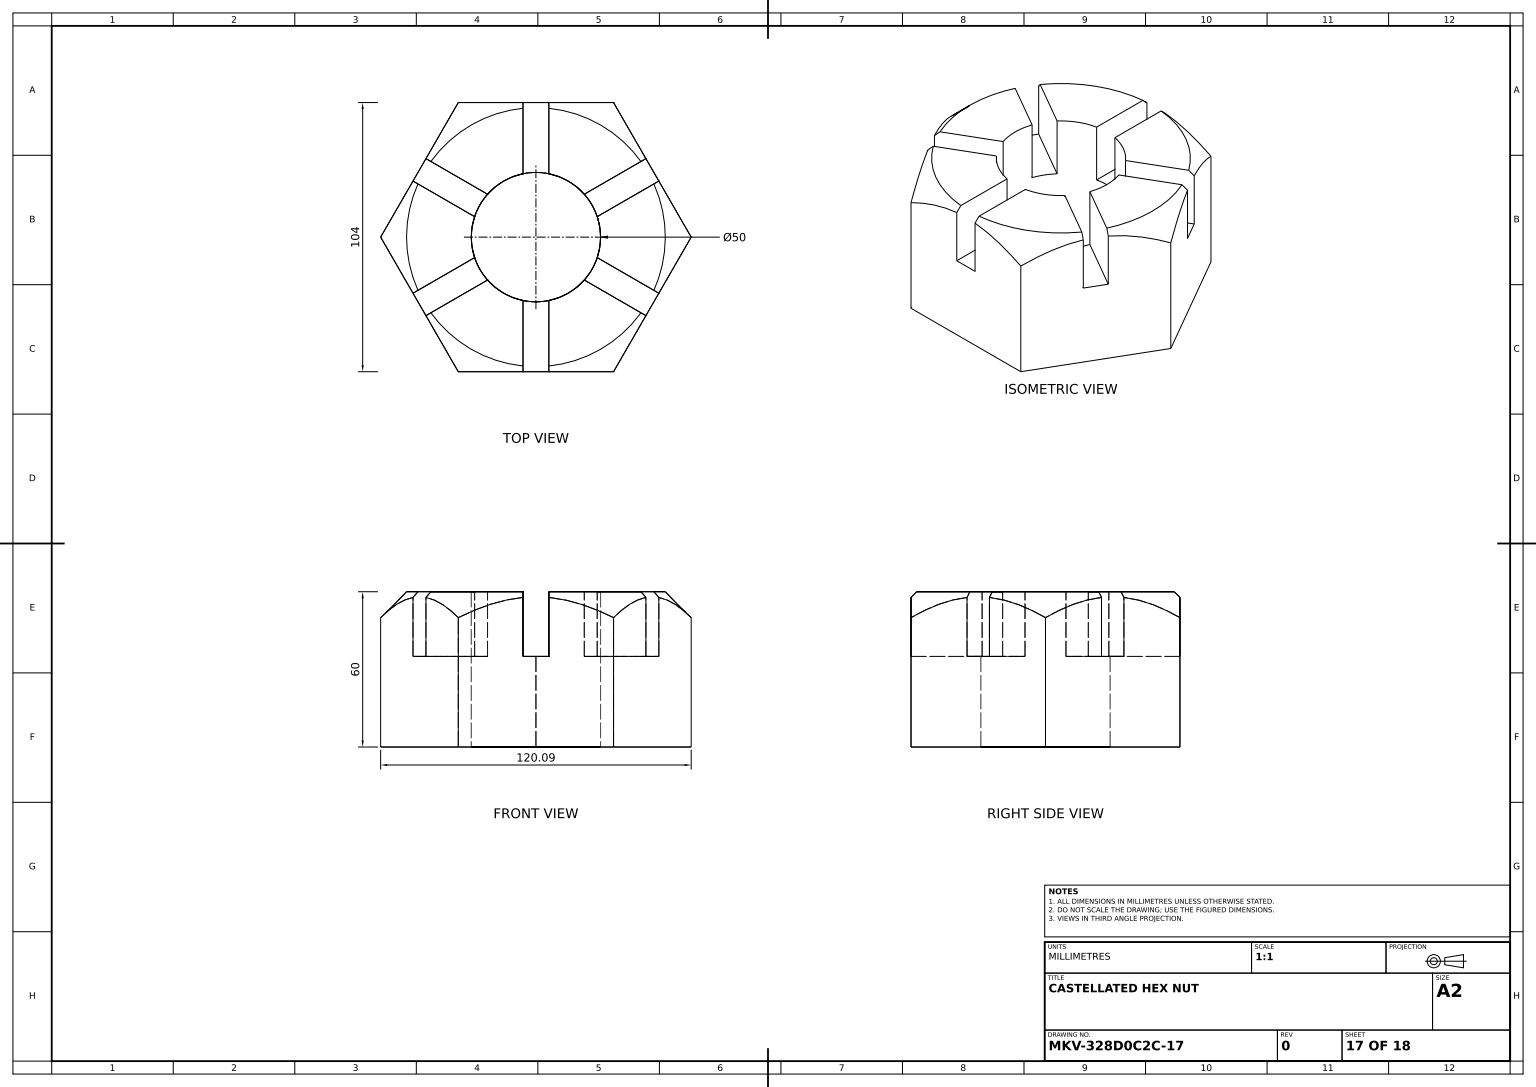
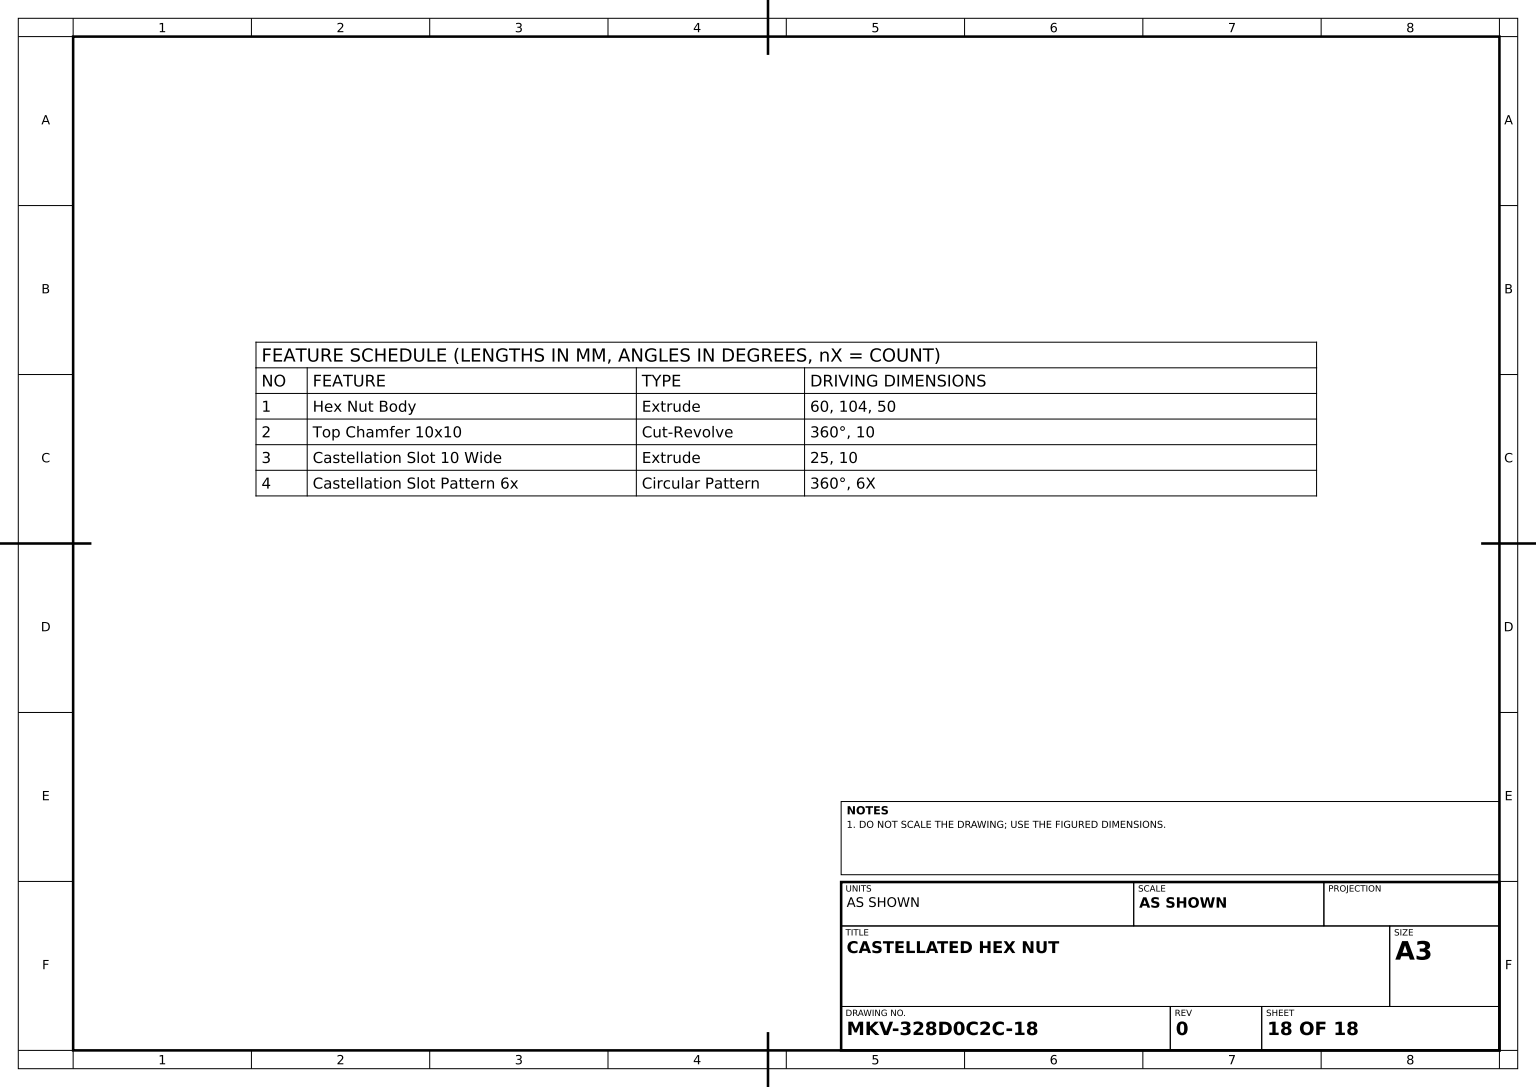
ISO-10303-21;
HEADER;
FILE_DESCRIPTION((''),'2;1');
FILE_NAME('','',(''),(''),'','','');
FILE_SCHEMA(('AUTOMOTIVE_DESIGN'));
ENDSEC;
DATA;
#1=APPLICATION_CONTEXT('');
#2=PRODUCT_CONTEXT('',#1,'mechanical');
#3=PRODUCT('','','',(#2));
#4=PRODUCT_DEFINITION_FORMATION('','',#3);
#5=PRODUCT_DEFINITION_CONTEXT('',#1,'design');
#6=PRODUCT_DEFINITION('','',#4,#5);
#7=PRODUCT_DEFINITION_SHAPE('','',#6);
#8=(LENGTH_UNIT()NAMED_UNIT(*)SI_UNIT(.MILLI.,.METRE.));
#9=(NAMED_UNIT(*)PLANE_ANGLE_UNIT()SI_UNIT($,.RADIAN.));
#10=(NAMED_UNIT(*)SI_UNIT($,.STERADIAN.)SOLID_ANGLE_UNIT());
#11=UNCERTAINTY_MEASURE_WITH_UNIT(LENGTH_MEASURE(1.E-05),#8,'distance_accuracy_value','');
#12=(GEOMETRIC_REPRESENTATION_CONTEXT(3)GLOBAL_UNCERTAINTY_ASSIGNED_CONTEXT((#11))GLOBAL_UNIT_ASSIGNED_CONTEXT((#8,#9,#10))REPRESENTATION_CONTEXT('',''));
#13=CARTESIAN_POINT('',(18.713203,-25.,16.577576));
#14=VERTEX_POINT('',#13);
#15=CARTESIAN_POINT('',(42.533321,-25.,30.330127));
#16=VERTEX_POINT('',#15);
#17=DIRECTION('',(0.866025404,0.,0.5));
#18=VECTOR('',#17,1000.);
#19=LINE('',#13,#18);
#20=EDGE_CURVE('',#14,#16,#19,.T.);
#21=ORIENTED_EDGE('',*,*,#20,.F.);
#22=CARTESIAN_POINT('',(18.713203,0.,16.577576));
#23=VERTEX_POINT('',#22);
#24=DIRECTION('',(0.,1.,0.));
#25=VECTOR('',#24,1000.);
#26=LINE('',#13,#25);
#27=EDGE_CURVE('',#14,#23,#26,.T.);
#28=ORIENTED_EDGE('',*,*,#27,.T.);
#29=CARTESIAN_POINT('',(40.622889,0.,29.227139));
#30=VERTEX_POINT('',#29);
#31=LINE('',#22,#18);
#32=EDGE_CURVE('',#23,#30,#31,.T.);
#33=ORIENTED_EDGE('',*,*,#32,.T.);
#34=CARTESIAN_POINT('',(42.533321,-2.195404,30.330127));
#35=VERTEX_POINT('',#34);
#36=CARTESIAN_POINT('',(41.896575,-1.463528,29.962501));
#37=CARTESIAN_POINT('',(41.259767,-0.731723,29.59484));
#38=B_SPLINE_CURVE_WITH_KNOTS('',3,(#34,#36,#37,#29),.UNSPECIFIED.,.F.,.F.,(4,4),(0.000000326,0.003112581),.UNSPECIFIED.);
#39=EDGE_CURVE('',#35,#30,#38,.T.);
#40=ORIENTED_EDGE('',*,*,#39,.F.);
#41=LINE('',#15,#25);
#42=EDGE_CURVE('',#16,#35,#41,.T.);
#43=ORIENTED_EDGE('',*,*,#42,.F.);
#44=EDGE_LOOP('',(#21,#28,#33,#40,#43));
#45=FACE_OUTER_BOUND('',#44,.T.);
#46=DIRECTION('',(-0.5,0.,0.866025404));
#47=AXIS2_PLACEMENT_3D('',#13,#46,#17);
#48=PLANE('',#47);
#49=ADVANCED_FACE('',(#45),#48,.F.);
#50=CARTESIAN_POINT('',(30.022214,-10.,52.));
#51=VERTEX_POINT('',#50);
#52=CARTESIAN_POINT('',(32.004718,-8.017496,48.566202));
#53=CARTESIAN_POINT('',(34.025227,-6.287322,45.066578));
#54=CARTESIAN_POINT('',(38.18079,-3.587487,37.868931));
#55=CARTESIAN_POINT('',(40.316146,-2.619826,34.170387));
#56=B_SPLINE_CURVE_WITH_KNOTS('',3,(#50,#52,#53,#54,#55,#34),.UNSPECIFIED.,.F.,.F.,(4,2,4),(0.000000254,0.013105191,0.026210128),.UNSPECIFIED.);
#57=EDGE_CURVE('',#51,#35,#56,.T.);
#58=ORIENTED_EDGE('',*,*,#57,.F.);
#59=CARTESIAN_POINT('',(30.022214,-60.,52.));
#60=VERTEX_POINT('',#59);
#61=LINE('',#59,#25);
#62=EDGE_CURVE('',#60,#51,#61,.T.);
#63=ORIENTED_EDGE('',*,*,#62,.F.);
#64=CARTESIAN_POINT('',(60.044428,-60.,0.));
#65=VERTEX_POINT('',#64);
#66=DIRECTION('',(0.5,0.,-0.866025404));
#67=VECTOR('',#66,1000.);
#68=LINE('',#59,#67);
#69=EDGE_CURVE('',#60,#65,#68,.T.);
#70=ORIENTED_EDGE('',*,*,#69,.T.);
#71=CARTESIAN_POINT('',(60.044428,-10.,0.));
#72=VERTEX_POINT('',#71);
#73=LINE('',#64,#25);
#74=EDGE_CURVE('',#65,#72,#73,.T.);
#75=ORIENTED_EDGE('',*,*,#74,.T.);
#76=CARTESIAN_POINT('',(47.533321,-2.195404,21.669873));
#77=VERTEX_POINT('',#76);
#78=CARTESIAN_POINT('',(48.617849,-2.403009,19.791415));
#79=CARTESIAN_POINT('',(49.694995,-2.743391,17.925744));
#80=CARTESIAN_POINT('',(51.300659,-3.434777,15.144652));
#81=CARTESIAN_POINT('',(51.834208,-3.695312,14.220518));
#82=CARTESIAN_POINT('',(52.898163,-4.272921,12.377694));
#83=CARTESIAN_POINT('',(53.428213,-4.589936,11.45962));
#84=CARTESIAN_POINT('',(55.000546,-5.610311,8.73626));
#85=CARTESIAN_POINT('',(56.029879,-6.385229,6.953403));
#86=CARTESIAN_POINT('',(58.058316,-8.086554,3.440047));
#87=CARTESIAN_POINT('',(59.057416,-9.012988,1.709555));
#88=B_SPLINE_CURVE_WITH_KNOTS('',3,(#76,#78,#79,#80,#81,#82,#83,#84,#85,#86,#87,#71),.UNSPECIFIED.,.F.,.F.,(4,2,2,2,2,4),(0.036078749,0.042565008,0.045808138,0.049051268,0.055537527,0.062023787),.UNSPECIFIED.);
#89=EDGE_CURVE('',#77,#72,#88,.T.);
#90=ORIENTED_EDGE('',*,*,#89,.F.);
#91=CARTESIAN_POINT('',(47.533321,-25.,21.669873));
#92=VERTEX_POINT('',#91);
#93=LINE('',#91,#25);
#94=EDGE_CURVE('',#92,#77,#93,.T.);
#95=ORIENTED_EDGE('',*,*,#94,.F.);
#96=LINE('',#91,#67);
#97=EDGE_CURVE('',#16,#92,#96,.T.);
#98=ORIENTED_EDGE('',*,*,#97,.F.);
#99=ORIENTED_EDGE('',*,*,#42,.T.);
#100=EDGE_LOOP('',(#58,#63,#70,#75,#90,#95,#98,#99));
#101=FACE_OUTER_BOUND('',#100,.T.);
#102=AXIS2_PLACEMENT_3D('',#59,#17,#66);
#103=PLANE('',#102);
#104=ADVANCED_FACE('',(#101),#103,.T.);
#105=CARTESIAN_POINT('',(23.713203,-25.,-7.917322));
#106=VERTEX_POINT('',#105);
#107=CARTESIAN_POINT('',(47.533321,-25.,-21.669873));
#108=VERTEX_POINT('',#107);
#109=DIRECTION('',(0.866025404,0.,-0.5));
#110=VECTOR('',#109,1000.);
#111=LINE('',#105,#110);
#112=EDGE_CURVE('',#106,#108,#111,.T.);
#113=ORIENTED_EDGE('',*,*,#112,.T.);
#114=CARTESIAN_POINT('',(42.533321,-25.,-30.330127));
#115=VERTEX_POINT('',#114);
#116=DIRECTION('',(-0.5,0.,-0.866025404));
#117=VECTOR('',#116,1000.);
#118=LINE('',#114,#117);
#119=EDGE_CURVE('',#108,#115,#118,.T.);
#120=ORIENTED_EDGE('',*,*,#119,.T.);
#121=CARTESIAN_POINT('',(18.713203,-25.,-16.577576));
#122=VERTEX_POINT('',#121);
#123=DIRECTION('',(-0.866025404,0.,0.5));
#124=VECTOR('',#123,1000.);
#125=LINE('',#121,#124);
#126=EDGE_CURVE('',#115,#122,#125,.T.);
#127=ORIENTED_EDGE('',*,*,#126,.T.);
#128=CARTESIAN_POINT('',(0.,-25.,0.));
#129=DIRECTION('',(0.,-1.,0.));
#130=AXIS2_PLACEMENT_3D('',#128,#129,#123);
#131=CIRCLE('',#130,25.);
#132=EDGE_CURVE('',#122,#106,#131,.T.);
#133=ORIENTED_EDGE('',*,*,#132,.T.);
#134=EDGE_LOOP('',(#113,#120,#127,#133));
#135=FACE_OUTER_BOUND('',#134,.T.);
#136=AXIS2_PLACEMENT_3D('',#128,#24,#123);
#137=PLANE('',#136);
#138=ADVANCED_FACE('',(#135),#137,.T.);
#139=CARTESIAN_POINT('',(-18.713203,0.,16.577576));
#140=VERTEX_POINT('',#139);
#141=CARTESIAN_POINT('',(-5.,0.,24.494897));
#142=VERTEX_POINT('',#141);
#143=CARTESIAN_POINT('',(0.,0.,0.));
#144=DIRECTION('',(0.,0.,1.));
#145=AXIS2_PLACEMENT_3D('',#143,#24,#144);
#146=CIRCLE('',#145,25.);
#147=EDGE_CURVE('',#140,#142,#146,.T.);
#148=ORIENTED_EDGE('',*,*,#147,.F.);
#149=CARTESIAN_POINT('',(-40.622889,0.,29.227139));
#150=VERTEX_POINT('',#149);
#151=LINE('',#139,#110);
#152=EDGE_CURVE('',#150,#140,#151,.T.);
#153=ORIENTED_EDGE('',*,*,#152,.F.);
#154=CARTESIAN_POINT('',(-5.,0.,49.794023));
#155=VERTEX_POINT('',#154);
#156=DIRECTION('',(0.,0.,-1.));
#157=AXIS2_PLACEMENT_3D('',#143,#129,#156);
#158=CIRCLE('',#157,50.044428);
#159=EDGE_CURVE('',#155,#150,#158,.T.);
#160=ORIENTED_EDGE('',*,*,#159,.F.);
#161=VECTOR('',#144,1000.);
#162=LINE('',#141,#161);
#163=EDGE_CURVE('',#142,#155,#162,.T.);
#164=ORIENTED_EDGE('',*,*,#163,.F.);
#165=EDGE_LOOP('',(#148,#153,#160,#164));
#166=FACE_OUTER_BOUND('',#165,.T.);
#167=PLANE('',#145);
#168=ADVANCED_FACE('',(#166),#167,.T.);
#169=CARTESIAN_POINT('',(23.713203,-25.,7.917322));
#170=VERTEX_POINT('',#169);
#171=CARTESIAN_POINT('',(23.713203,0.,7.917322));
#172=VERTEX_POINT('',#171);
#173=LINE('',#169,#25);
#174=EDGE_CURVE('',#170,#172,#173,.T.);
#175=ORIENTED_EDGE('',*,*,#174,.T.);
#176=CARTESIAN_POINT('',(23.713203,0.,-7.917322));
#177=VERTEX_POINT('',#176);
#178=EDGE_CURVE('',#172,#177,#146,.T.);
#179=ORIENTED_EDGE('',*,*,#178,.T.);
#180=LINE('',#105,#25);
#181=EDGE_CURVE('',#106,#177,#180,.T.);
#182=ORIENTED_EDGE('',*,*,#181,.F.);
#183=ORIENTED_EDGE('',*,*,#132,.F.);
#184=CARTESIAN_POINT('',(18.713203,0.,-16.577576));
#185=VERTEX_POINT('',#184);
#186=LINE('',#121,#25);
#187=EDGE_CURVE('',#122,#185,#186,.T.);
#188=ORIENTED_EDGE('',*,*,#187,.T.);
#189=CARTESIAN_POINT('',(5.,0.,-24.494897));
#190=VERTEX_POINT('',#189);
#191=EDGE_CURVE('',#185,#190,#146,.T.);
#192=ORIENTED_EDGE('',*,*,#191,.T.);
#193=CARTESIAN_POINT('',(5.,-25.,-24.494897));
#194=VERTEX_POINT('',#193);
#195=LINE('',#193,#25);
#196=EDGE_CURVE('',#194,#190,#195,.T.);
#197=ORIENTED_EDGE('',*,*,#196,.F.);
#198=CARTESIAN_POINT('',(0.,-25.,-25.));
#199=VERTEX_POINT('',#198);
#200=AXIS2_PLACEMENT_3D('',#128,#129,#144);
#201=CIRCLE('',#200,25.);
#202=EDGE_CURVE('',#199,#194,#201,.T.);
#203=ORIENTED_EDGE('',*,*,#202,.F.);
#204=CARTESIAN_POINT('',(0.,-60.,-25.));
#205=VERTEX_POINT('',#204);
#206=LINE('',#204,#25);
#207=EDGE_CURVE('',#205,#199,#206,.T.);
#208=ORIENTED_EDGE('',*,*,#207,.F.);
#209=CARTESIAN_POINT('',(0.,-60.,25.));
#210=VERTEX_POINT('',#209);
#211=CARTESIAN_POINT('',(0.,-60.,0.));
#212=AXIS2_PLACEMENT_3D('',#211,#24,#144);
#213=CIRCLE('',#212,25.);
#214=EDGE_CURVE('',#210,#205,#213,.T.);
#215=ORIENTED_EDGE('',*,*,#214,.F.);
#216=CARTESIAN_POINT('',(0.,-25.,25.));
#217=VERTEX_POINT('',#216);
#218=LINE('',#209,#25);
#219=EDGE_CURVE('',#210,#217,#218,.T.);
#220=ORIENTED_EDGE('',*,*,#219,.T.);
#221=CARTESIAN_POINT('',(5.,-25.,24.494897));
#222=VERTEX_POINT('',#221);
#223=AXIS2_PLACEMENT_3D('',#128,#129,#156);
#224=CIRCLE('',#223,25.);
#225=EDGE_CURVE('',#222,#217,#224,.T.);
#226=ORIENTED_EDGE('',*,*,#225,.F.);
#227=CARTESIAN_POINT('',(5.,0.,24.494897));
#228=VERTEX_POINT('',#227);
#229=LINE('',#221,#25);
#230=EDGE_CURVE('',#222,#228,#229,.T.);
#231=ORIENTED_EDGE('',*,*,#230,.T.);
#232=EDGE_CURVE('',#228,#23,#146,.T.);
#233=ORIENTED_EDGE('',*,*,#232,.T.);
#234=ORIENTED_EDGE('',*,*,#27,.F.);
#235=DIRECTION('',(-0.866025404,0.,-0.5));
#236=AXIS2_PLACEMENT_3D('',#128,#129,#235);
#237=CIRCLE('',#236,25.);
#238=EDGE_CURVE('',#170,#14,#237,.T.);
#239=ORIENTED_EDGE('',*,*,#238,.F.);
#240=EDGE_LOOP('',(#175,#179,#182,#183,#188,#192,#197,#203,#208,#215,#220,#226,#231,#233,#234,#239));
#241=FACE_OUTER_BOUND('',#240,.T.);
#242=CYLINDRICAL_SURFACE('',#212,25.);
#243=ADVANCED_FACE('',(#241),#242,.F.);
#244=CARTESIAN_POINT('',(-23.713203,0.,-7.917322));
#245=VERTEX_POINT('',#244);
#246=CARTESIAN_POINT('',(-23.713203,0.,7.917322));
#247=VERTEX_POINT('',#246);
#248=EDGE_CURVE('',#245,#247,#146,.T.);
#249=ORIENTED_EDGE('',*,*,#248,.F.);
#250=CARTESIAN_POINT('',(-45.622889,0.,-20.566885));
#251=VERTEX_POINT('',#250);
#252=LINE('',#244,#18);
#253=EDGE_CURVE('',#251,#245,#252,.T.);
#254=ORIENTED_EDGE('',*,*,#253,.F.);
#255=CARTESIAN_POINT('',(-45.622889,0.,20.566885));
#256=VERTEX_POINT('',#255);
#257=EDGE_CURVE('',#256,#251,#158,.T.);
#258=ORIENTED_EDGE('',*,*,#257,.F.);
#259=LINE('',#246,#124);
#260=EDGE_CURVE('',#247,#256,#259,.T.);
#261=ORIENTED_EDGE('',*,*,#260,.F.);
#262=EDGE_LOOP('',(#249,#254,#258,#261));
#263=FACE_OUTER_BOUND('',#262,.T.);
#264=ADVANCED_FACE('',(#263),#167,.T.);
#265=CARTESIAN_POINT('',(5.,0.,-49.794023));
#266=VERTEX_POINT('',#265);
#267=CARTESIAN_POINT('',(40.622889,0.,-29.227139));
#268=VERTEX_POINT('',#267);
#269=EDGE_CURVE('',#266,#268,#158,.T.);
#270=ORIENTED_EDGE('',*,*,#269,.F.);
#271=VECTOR('',#156,1000.);
#272=LINE('',#189,#271);
#273=EDGE_CURVE('',#190,#266,#272,.T.);
#274=ORIENTED_EDGE('',*,*,#273,.F.);
#275=ORIENTED_EDGE('',*,*,#191,.F.);
#276=LINE('',#184,#124);
#277=EDGE_CURVE('',#268,#185,#276,.T.);
#278=ORIENTED_EDGE('',*,*,#277,.F.);
#279=EDGE_LOOP('',(#270,#274,#275,#278));
#280=FACE_OUTER_BOUND('',#279,.T.);
#281=ADVANCED_FACE('',(#280),#167,.T.);
#282=CARTESIAN_POINT('',(47.533321,-2.195404,-21.669873));
#283=VERTEX_POINT('',#282);
#284=LINE('',#107,#25);
#285=EDGE_CURVE('',#108,#283,#284,.T.);
#286=ORIENTED_EDGE('',*,*,#285,.F.);
#287=ORIENTED_EDGE('',*,*,#112,.F.);
#288=ORIENTED_EDGE('',*,*,#181,.T.);
#289=CARTESIAN_POINT('',(45.622889,0.,-20.566885));
#290=VERTEX_POINT('',#289);
#291=LINE('',#176,#110);
#292=EDGE_CURVE('',#177,#290,#291,.T.);
#293=ORIENTED_EDGE('',*,*,#292,.T.);
#294=CARTESIAN_POINT('',(46.896575,-1.463528,-21.302247));
#295=CARTESIAN_POINT('',(46.259767,-0.731723,-20.934586));
#296=B_SPLINE_CURVE_WITH_KNOTS('',3,(#282,#294,#295,#289),.UNSPECIFIED.,.F.,.F.,(4,4),(0.000000326,0.003112581),.UNSPECIFIED.);
#297=EDGE_CURVE('',#283,#290,#296,.T.);
#298=ORIENTED_EDGE('',*,*,#297,.F.);
#299=EDGE_LOOP('',(#286,#287,#288,#293,#298));
#300=FACE_OUTER_BOUND('',#299,.T.);
#301=DIRECTION('',(0.5,0.,0.866025404));
#302=AXIS2_PLACEMENT_3D('',#105,#301,#109);
#303=PLANE('',#302);
#304=ADVANCED_FACE('',(#300),#303,.F.);
#305=CARTESIAN_POINT('',(5.,0.,49.794023));
#306=VERTEX_POINT('',#305);
#307=CARTESIAN_POINT('',(5.,-2.195404,52.));
#308=VERTEX_POINT('',#307);
#309=CARTESIAN_POINT('',(5.,-0.731723,50.529427));
#310=CARTESIAN_POINT('',(5.,-1.463528,51.264749));
#311=B_SPLINE_CURVE_WITH_KNOTS('',3,(#305,#309,#310,#307),.UNSPECIFIED.,.F.,.F.,(4,4),(0.041644919,0.044757161),.UNSPECIFIED.);
#312=EDGE_CURVE('',#306,#308,#311,.T.);
#313=ORIENTED_EDGE('',*,*,#312,.T.);
#314=CARTESIAN_POINT('',(9.390566,-2.615635,52.));
#315=CARTESIAN_POINT('',(13.657016,-3.573826,52.));
#316=CARTESIAN_POINT('',(18.875839,-5.266714,52.));
#317=CARTESIAN_POINT('',(19.913896,-5.630031,52.));
#318=CARTESIAN_POINT('',(21.979581,-6.401866,52.));
#319=CARTESIAN_POINT('',(23.009249,-6.811255,52.));
#320=CARTESIAN_POINT('',(26.068458,-8.094517,52.));
#321=CARTESIAN_POINT('',(28.062721,-9.020253,52.));
#322=B_SPLINE_CURVE_WITH_KNOTS('',3,(#307,#314,#315,#316,#317,#318,#319,#320,#321,#50),.UNSPECIFIED.,.F.,.F.,(4,2,2,2,4),(0.112045409,0.125191759,0.128478347,0.131764934,0.138338109),.UNSPECIFIED.);
#323=EDGE_CURVE('',#308,#51,#322,.T.);
#324=ORIENTED_EDGE('',*,*,#323,.T.);
#325=ORIENTED_EDGE('',*,*,#57,.T.);
#326=ORIENTED_EDGE('',*,*,#39,.T.);
#327=EDGE_CURVE('',#30,#306,#158,.T.);
#328=ORIENTED_EDGE('',*,*,#327,.T.);
#329=EDGE_LOOP('',(#313,#324,#325,#326,#328));
#330=FACE_OUTER_BOUND('',#329,.T.);
#331=CONICAL_SURFACE('',#157,50.044427996,0.785398163);
#332=ADVANCED_FACE('',(#330),#331,.T.);
#333=CARTESIAN_POINT('',(-47.533321,-2.195404,21.669873));
#334=VERTEX_POINT('',#333);
#335=CARTESIAN_POINT('',(-46.896575,-1.463528,21.302247));
#336=CARTESIAN_POINT('',(-46.259767,-0.731723,20.934586));
#337=B_SPLINE_CURVE_WITH_KNOTS('',3,(#333,#335,#336,#255),.UNSPECIFIED.,.F.,.F.,(4,4),(0.000000326,0.003112581),.UNSPECIFIED.);
#338=EDGE_CURVE('',#334,#256,#337,.T.);
#339=ORIENTED_EDGE('',*,*,#338,.T.);
#340=ORIENTED_EDGE('',*,*,#257,.T.);
#341=CARTESIAN_POINT('',(-47.533321,-2.195404,-21.669873));
#342=VERTEX_POINT('',#341);
#343=CARTESIAN_POINT('',(-46.259767,-0.731723,-20.934586));
#344=CARTESIAN_POINT('',(-46.896575,-1.463528,-21.302247));
#345=B_SPLINE_CURVE_WITH_KNOTS('',3,(#250,#343,#344,#341),.UNSPECIFIED.,.F.,.F.,(4,4),(0.000000284,0.003112538),.UNSPECIFIED.);
#346=EDGE_CURVE('',#251,#342,#345,.T.);
#347=ORIENTED_EDGE('',*,*,#346,.T.);
#348=CARTESIAN_POINT('',(-60.044428,-10.,0.));
#349=VERTEX_POINT('',#348);
#350=CARTESIAN_POINT('',(-48.617849,-2.403009,-19.791415));
#351=CARTESIAN_POINT('',(-49.694995,-2.743391,-17.925744));
#352=CARTESIAN_POINT('',(-51.300659,-3.434777,-15.144652));
#353=CARTESIAN_POINT('',(-51.834208,-3.695312,-14.220518));
#354=CARTESIAN_POINT('',(-52.898163,-4.272921,-12.377694));
#355=CARTESIAN_POINT('',(-53.428213,-4.589936,-11.45962));
#356=CARTESIAN_POINT('',(-55.000546,-5.610311,-8.73626));
#357=CARTESIAN_POINT('',(-56.029879,-6.385229,-6.953403));
#358=CARTESIAN_POINT('',(-58.058316,-8.086554,-3.440047));
#359=CARTESIAN_POINT('',(-59.057416,-9.012988,-1.709555));
#360=B_SPLINE_CURVE_WITH_KNOTS('',3,(#341,#350,#351,#352,#353,#354,#355,#356,#357,#358,#359,#348),.UNSPECIFIED.,.F.,.F.,(4,2,2,2,2,4),(0.036078749,0.042565008,0.045808138,0.049051268,0.055537527,0.062023787),.UNSPECIFIED.);
#361=EDGE_CURVE('',#342,#349,#360,.T.);
#362=ORIENTED_EDGE('',*,*,#361,.T.);
#363=CARTESIAN_POINT('',(-58.061924,-8.017496,3.433798));
#364=CARTESIAN_POINT('',(-56.041415,-6.287322,6.933422));
#365=CARTESIAN_POINT('',(-51.885852,-3.587487,14.131069));
#366=CARTESIAN_POINT('',(-49.750496,-2.619826,17.829613));
#367=B_SPLINE_CURVE_WITH_KNOTS('',3,(#348,#363,#364,#365,#366,#333),.UNSPECIFIED.,.F.,.F.,(4,2,4),(0.000000254,0.013105191,0.026210128),.UNSPECIFIED.);
#368=EDGE_CURVE('',#349,#334,#367,.T.);
#369=ORIENTED_EDGE('',*,*,#368,.T.);
#370=EDGE_LOOP('',(#339,#340,#347,#362,#369));
#371=FACE_OUTER_BOUND('',#370,.T.);
#372=ADVANCED_FACE('',(#371),#331,.T.);
#373=CARTESIAN_POINT('',(-5.,-25.,52.));
#374=VERTEX_POINT('',#373);
#375=CARTESIAN_POINT('',(-5.,-2.195404,52.));
#376=VERTEX_POINT('',#375);
#377=LINE('',#373,#25);
#378=EDGE_CURVE('',#374,#376,#377,.T.);
#379=ORIENTED_EDGE('',*,*,#378,.T.);
#380=CARTESIAN_POINT('',(-30.022214,-10.,52.));
#381=VERTEX_POINT('',#380);
#382=CARTESIAN_POINT('',(-28.066253,-9.02202,52.));
#383=CARTESIAN_POINT('',(-26.078269,-8.099222,52.));
#384=CARTESIAN_POINT('',(-23.034477,-6.821547,52.));
#385=CARTESIAN_POINT('',(-22.009536,-6.413479,52.));
#386=CARTESIAN_POINT('',(-19.936107,-5.637921,52.));
#387=CARTESIAN_POINT('',(-18.886961,-5.270393,52.));
#388=CARTESIAN_POINT('',(-13.633075,-3.565779,52.));
#389=CARTESIAN_POINT('',(-9.3613,-2.612834,52.));
#390=B_SPLINE_CURVE_WITH_KNOTS('',3,(#380,#382,#383,#384,#385,#386,#387,#388,#389,#375),.UNSPECIFIED.,.F.,.F.,(4,2,2,2,4),(0.075775664,0.082357953,0.085649098,0.088940243,0.102104821),.UNSPECIFIED.);
#391=EDGE_CURVE('',#381,#376,#390,.T.);
#392=ORIENTED_EDGE('',*,*,#391,.F.);
#393=CARTESIAN_POINT('',(-30.022214,-60.,52.));
#394=VERTEX_POINT('',#393);
#395=LINE('',#393,#25);
#396=EDGE_CURVE('',#394,#381,#395,.T.);
#397=ORIENTED_EDGE('',*,*,#396,.F.);
#398=DIRECTION('',(1.,0.,0.));
#399=VECTOR('',#398,1000.);
#400=LINE('',#393,#399);
#401=EDGE_CURVE('',#394,#60,#400,.T.);
#402=ORIENTED_EDGE('',*,*,#401,.T.);
#403=ORIENTED_EDGE('',*,*,#62,.T.);
#404=ORIENTED_EDGE('',*,*,#323,.F.);
#405=CARTESIAN_POINT('',(5.,-25.,52.));
#406=VERTEX_POINT('',#405);
#407=LINE('',#405,#25);
#408=EDGE_CURVE('',#406,#308,#407,.T.);
#409=ORIENTED_EDGE('',*,*,#408,.F.);
#410=LINE('',#405,#399);
#411=EDGE_CURVE('',#374,#406,#410,.T.);
#412=ORIENTED_EDGE('',*,*,#411,.F.);
#413=EDGE_LOOP('',(#379,#392,#397,#402,#403,#404,#409,#412));
#414=FACE_OUTER_BOUND('',#413,.T.);
#415=AXIS2_PLACEMENT_3D('',#393,#144,#398);
#416=PLANE('',#415);
#417=ADVANCED_FACE('',(#414),#416,.T.);
#418=CARTESIAN_POINT('',(-47.533321,-25.,-21.669873));
#419=VERTEX_POINT('',#418);
#420=LINE('',#418,#25);
#421=EDGE_CURVE('',#419,#342,#420,.T.);
#422=ORIENTED_EDGE('',*,*,#421,.T.);
#423=ORIENTED_EDGE('',*,*,#346,.F.);
#424=ORIENTED_EDGE('',*,*,#253,.T.);
#425=CARTESIAN_POINT('',(-23.713203,-25.,-7.917322));
#426=VERTEX_POINT('',#425);
#427=LINE('',#425,#25);
#428=EDGE_CURVE('',#426,#245,#427,.T.);
#429=ORIENTED_EDGE('',*,*,#428,.F.);
#430=LINE('',#425,#18);
#431=EDGE_CURVE('',#419,#426,#430,.T.);
#432=ORIENTED_EDGE('',*,*,#431,.F.);
#433=EDGE_LOOP('',(#422,#423,#424,#429,#432));
#434=FACE_OUTER_BOUND('',#433,.T.);
#435=AXIS2_PLACEMENT_3D('',#425,#46,#17);
#436=PLANE('',#435);
#437=ADVANCED_FACE('',(#434),#436,.F.);
#438=CARTESIAN_POINT('',(-5.,-1.463528,51.264749));
#439=CARTESIAN_POINT('',(-5.,-0.731723,50.529426));
#440=B_SPLINE_CURVE_WITH_KNOTS('',3,(#375,#438,#439,#154),.UNSPECIFIED.,.F.,.F.,(4,4),(0.04132844,0.044440691),.UNSPECIFIED.);
#441=EDGE_CURVE('',#376,#155,#440,.T.);
#442=ORIENTED_EDGE('',*,*,#441,.T.);
#443=ORIENTED_EDGE('',*,*,#159,.T.);
#444=CARTESIAN_POINT('',(-42.533321,-2.195404,30.330127));
#445=VERTEX_POINT('',#444);
#446=CARTESIAN_POINT('',(-41.259767,-0.731723,29.59484));
#447=CARTESIAN_POINT('',(-41.896575,-1.463528,29.962501));
#448=B_SPLINE_CURVE_WITH_KNOTS('',3,(#149,#446,#447,#444),.UNSPECIFIED.,.F.,.F.,(4,4),(0.000000284,0.003112538),.UNSPECIFIED.);
#449=EDGE_CURVE('',#150,#445,#448,.T.);
#450=ORIENTED_EDGE('',*,*,#449,.T.);
#451=CARTESIAN_POINT('',(-41.448793,-2.403009,32.208585));
#452=CARTESIAN_POINT('',(-40.371647,-2.743391,34.074256));
#453=CARTESIAN_POINT('',(-38.765983,-3.434777,36.855348));
#454=CARTESIAN_POINT('',(-38.232434,-3.695312,37.779482));
#455=CARTESIAN_POINT('',(-37.168479,-4.272921,39.622306));
#456=CARTESIAN_POINT('',(-36.638429,-4.589936,40.54038));
#457=CARTESIAN_POINT('',(-35.066096,-5.610311,43.26374));
#458=CARTESIAN_POINT('',(-34.036763,-6.385229,45.046597));
#459=CARTESIAN_POINT('',(-32.008326,-8.086554,48.559953));
#460=CARTESIAN_POINT('',(-31.009226,-9.012988,50.290445));
#461=B_SPLINE_CURVE_WITH_KNOTS('',3,(#444,#451,#452,#453,#454,#455,#456,#457,#458,#459,#460,#380),.UNSPECIFIED.,.F.,.F.,(4,2,2,2,2,4),(0.036078749,0.042565008,0.045808138,0.049051268,0.055537527,0.062023787),.UNSPECIFIED.);
#462=EDGE_CURVE('',#445,#381,#461,.T.);
#463=ORIENTED_EDGE('',*,*,#462,.T.);
#464=ORIENTED_EDGE('',*,*,#391,.T.);
#465=EDGE_LOOP('',(#442,#443,#450,#463,#464));
#466=FACE_OUTER_BOUND('',#465,.T.);
#467=ADVANCED_FACE('',(#466),#331,.T.);
#468=CARTESIAN_POINT('',(5.,-2.195404,-52.));
#469=VERTEX_POINT('',#468);
#470=CARTESIAN_POINT('',(5.,-1.463528,-51.264749));
#471=CARTESIAN_POINT('',(5.,-0.731723,-50.529426));
#472=B_SPLINE_CURVE_WITH_KNOTS('',3,(#468,#470,#471,#265),.UNSPECIFIED.,.F.,.F.,(4,4),(0.04132844,0.044440691),.UNSPECIFIED.);
#473=EDGE_CURVE('',#469,#266,#472,.T.);
#474=ORIENTED_EDGE('',*,*,#473,.F.);
#475=CARTESIAN_POINT('',(5.,-25.,-52.));
#476=VERTEX_POINT('',#475);
#477=LINE('',#475,#25);
#478=EDGE_CURVE('',#476,#469,#477,.T.);
#479=ORIENTED_EDGE('',*,*,#478,.F.);
#480=LINE('',#193,#271);
#481=EDGE_CURVE('',#194,#476,#480,.T.);
#482=ORIENTED_EDGE('',*,*,#481,.F.);
#483=ORIENTED_EDGE('',*,*,#196,.T.);
#484=ORIENTED_EDGE('',*,*,#273,.T.);
#485=EDGE_LOOP('',(#474,#479,#482,#483,#484));
#486=FACE_OUTER_BOUND('',#485,.T.);
#487=AXIS2_PLACEMENT_3D('',#193,#398,#156);
#488=PLANE('',#487);
#489=ADVANCED_FACE('',(#486),#488,.F.);
#490=ORIENTED_EDGE('',*,*,#292,.F.);
#491=ORIENTED_EDGE('',*,*,#178,.F.);
#492=CARTESIAN_POINT('',(45.622889,0.,20.566885));
#493=VERTEX_POINT('',#492);
#494=VECTOR('',#235,1000.);
#495=LINE('',#171,#494);
#496=EDGE_CURVE('',#493,#172,#495,.T.);
#497=ORIENTED_EDGE('',*,*,#496,.F.);
#498=EDGE_CURVE('',#290,#493,#158,.T.);
#499=ORIENTED_EDGE('',*,*,#498,.F.);
#500=EDGE_LOOP('',(#490,#491,#497,#499));
#501=FACE_OUTER_BOUND('',#500,.T.);
#502=ADVANCED_FACE('',(#501),#167,.T.);
#503=ORIENTED_EDGE('',*,*,#260,.T.);
#504=ORIENTED_EDGE('',*,*,#338,.F.);
#505=CARTESIAN_POINT('',(-47.533321,-25.,21.669873));
#506=VERTEX_POINT('',#505);
#507=LINE('',#505,#25);
#508=EDGE_CURVE('',#506,#334,#507,.T.);
#509=ORIENTED_EDGE('',*,*,#508,.F.);
#510=CARTESIAN_POINT('',(-23.713203,-25.,7.917322));
#511=VERTEX_POINT('',#510);
#512=LINE('',#510,#124);
#513=EDGE_CURVE('',#511,#506,#512,.T.);
#514=ORIENTED_EDGE('',*,*,#513,.F.);
#515=LINE('',#510,#25);
#516=EDGE_CURVE('',#511,#247,#515,.T.);
#517=ORIENTED_EDGE('',*,*,#516,.T.);
#518=EDGE_LOOP('',(#503,#504,#509,#514,#517));
#519=FACE_OUTER_BOUND('',#518,.T.);
#520=AXIS2_PLACEMENT_3D('',#510,#116,#123);
#521=PLANE('',#520);
#522=ADVANCED_FACE('',(#519),#521,.F.);
#523=CARTESIAN_POINT('',(-5.,-25.,24.494897));
#524=VERTEX_POINT('',#523);
#525=EDGE_CURVE('',#217,#524,#224,.T.);
#526=ORIENTED_EDGE('',*,*,#525,.F.);
#527=ORIENTED_EDGE('',*,*,#219,.F.);
#528=EDGE_CURVE('',#205,#210,#213,.T.);
#529=ORIENTED_EDGE('',*,*,#528,.F.);
#530=ORIENTED_EDGE('',*,*,#207,.T.);
#531=CARTESIAN_POINT('',(-5.,-25.,-24.494897));
#532=VERTEX_POINT('',#531);
#533=EDGE_CURVE('',#532,#199,#201,.T.);
#534=ORIENTED_EDGE('',*,*,#533,.F.);
#535=CARTESIAN_POINT('',(-5.,0.,-24.494897));
#536=VERTEX_POINT('',#535);
#537=LINE('',#531,#25);
#538=EDGE_CURVE('',#532,#536,#537,.T.);
#539=ORIENTED_EDGE('',*,*,#538,.T.);
#540=CARTESIAN_POINT('',(-18.713203,0.,-16.577576));
#541=VERTEX_POINT('',#540);
#542=EDGE_CURVE('',#536,#541,#146,.T.);
#543=ORIENTED_EDGE('',*,*,#542,.T.);
#544=CARTESIAN_POINT('',(-18.713203,-25.,-16.577576));
#545=VERTEX_POINT('',#544);
#546=LINE('',#544,#25);
#547=EDGE_CURVE('',#545,#541,#546,.T.);
#548=ORIENTED_EDGE('',*,*,#547,.F.);
#549=AXIS2_PLACEMENT_3D('',#128,#129,#17);
#550=CIRCLE('',#549,25.);
#551=EDGE_CURVE('',#426,#545,#550,.T.);
#552=ORIENTED_EDGE('',*,*,#551,.F.);
#553=ORIENTED_EDGE('',*,*,#428,.T.);
#554=ORIENTED_EDGE('',*,*,#248,.T.);
#555=ORIENTED_EDGE('',*,*,#516,.F.);
#556=CARTESIAN_POINT('',(-18.713203,-25.,16.577576));
#557=VERTEX_POINT('',#556);
#558=AXIS2_PLACEMENT_3D('',#128,#129,#109);
#559=CIRCLE('',#558,25.);
#560=EDGE_CURVE('',#557,#511,#559,.T.);
#561=ORIENTED_EDGE('',*,*,#560,.F.);
#562=LINE('',#556,#25);
#563=EDGE_CURVE('',#557,#140,#562,.T.);
#564=ORIENTED_EDGE('',*,*,#563,.T.);
#565=ORIENTED_EDGE('',*,*,#147,.T.);
#566=LINE('',#523,#25);
#567=EDGE_CURVE('',#524,#142,#566,.T.);
#568=ORIENTED_EDGE('',*,*,#567,.F.);
#569=EDGE_LOOP('',(#526,#527,#529,#530,#534,#539,#543,#548,#552,#553,#554,#555,#561,#564,#565,#568));
#570=FACE_OUTER_BOUND('',#569,.T.);
#571=ADVANCED_FACE('',(#570),#242,.F.);
#572=ORIENTED_EDGE('',*,*,#401,.F.);
#573=CARTESIAN_POINT('',(-60.044428,-60.,0.));
#574=VERTEX_POINT('',#573);
#575=VECTOR('',#301,1000.);
#576=LINE('',#573,#575);
#577=EDGE_CURVE('',#574,#394,#576,.T.);
#578=ORIENTED_EDGE('',*,*,#577,.F.);
#579=CARTESIAN_POINT('',(-30.022214,-60.,-52.));
#580=VERTEX_POINT('',#579);
#581=VECTOR('',#46,1000.);
#582=LINE('',#579,#581);
#583=EDGE_CURVE('',#580,#574,#582,.T.);
#584=ORIENTED_EDGE('',*,*,#583,.F.);
#585=CARTESIAN_POINT('',(30.022214,-60.,-52.));
#586=VERTEX_POINT('',#585);
#587=DIRECTION('',(-1.,0.,0.));
#588=VECTOR('',#587,1000.);
#589=LINE('',#585,#588);
#590=EDGE_CURVE('',#586,#580,#589,.T.);
#591=ORIENTED_EDGE('',*,*,#590,.F.);
#592=LINE('',#64,#117);
#593=EDGE_CURVE('',#65,#586,#592,.T.);
#594=ORIENTED_EDGE('',*,*,#593,.F.);
#595=ORIENTED_EDGE('',*,*,#69,.F.);
#596=EDGE_LOOP('',(#572,#578,#584,#591,#594,#595));
#597=FACE_OUTER_BOUND('',#596,.T.);
#598=ORIENTED_EDGE('',*,*,#214,.T.);
#599=ORIENTED_EDGE('',*,*,#528,.T.);
#600=EDGE_LOOP('',(#598,#599));
#601=FACE_BOUND('',#600,.T.);
#602=PLANE('',#212);
#603=ADVANCED_FACE('',(#597,#601),#602,.F.);
#604=CARTESIAN_POINT('',(-5.,-25.,-52.));
#605=VERTEX_POINT('',#604);
#606=CARTESIAN_POINT('',(-5.,-2.195404,-52.));
#607=VERTEX_POINT('',#606);
#608=LINE('',#604,#25);
#609=EDGE_CURVE('',#605,#607,#608,.T.);
#610=ORIENTED_EDGE('',*,*,#609,.F.);
#611=LINE('',#604,#588);
#612=EDGE_CURVE('',#476,#605,#611,.T.);
#613=ORIENTED_EDGE('',*,*,#612,.F.);
#614=ORIENTED_EDGE('',*,*,#478,.T.);
#615=CARTESIAN_POINT('',(30.022214,-10.,-52.));
#616=VERTEX_POINT('',#615);
#617=CARTESIAN_POINT('',(28.066253,-9.02202,-52.));
#618=CARTESIAN_POINT('',(26.078269,-8.099222,-52.));
#619=CARTESIAN_POINT('',(23.034477,-6.821547,-52.));
#620=CARTESIAN_POINT('',(22.009536,-6.413479,-52.));
#621=CARTESIAN_POINT('',(19.936107,-5.637921,-52.));
#622=CARTESIAN_POINT('',(18.886961,-5.270393,-52.));
#623=CARTESIAN_POINT('',(13.633075,-3.565779,-52.));
#624=CARTESIAN_POINT('',(9.3613,-2.612834,-52.));
#625=B_SPLINE_CURVE_WITH_KNOTS('',3,(#615,#617,#618,#619,#620,#621,#622,#623,#624,#468),.UNSPECIFIED.,.F.,.F.,(4,2,2,2,4),(0.075775664,0.082357953,0.085649098,0.088940243,0.102104821),.UNSPECIFIED.);
#626=EDGE_CURVE('',#616,#469,#625,.T.);
#627=ORIENTED_EDGE('',*,*,#626,.F.);
#628=LINE('',#585,#25);
#629=EDGE_CURVE('',#586,#616,#628,.T.);
#630=ORIENTED_EDGE('',*,*,#629,.F.);
#631=ORIENTED_EDGE('',*,*,#590,.T.);
#632=CARTESIAN_POINT('',(-30.022214,-10.,-52.));
#633=VERTEX_POINT('',#632);
#634=LINE('',#579,#25);
#635=EDGE_CURVE('',#580,#633,#634,.T.);
#636=ORIENTED_EDGE('',*,*,#635,.T.);
#637=CARTESIAN_POINT('',(-9.390566,-2.615635,-52.));
#638=CARTESIAN_POINT('',(-13.657016,-3.573826,-52.));
#639=CARTESIAN_POINT('',(-18.875839,-5.266714,-52.));
#640=CARTESIAN_POINT('',(-19.913896,-5.630031,-52.));
#641=CARTESIAN_POINT('',(-21.979581,-6.401866,-52.));
#642=CARTESIAN_POINT('',(-23.009249,-6.811255,-52.));
#643=CARTESIAN_POINT('',(-26.068458,-8.094517,-52.));
#644=CARTESIAN_POINT('',(-28.062721,-9.020253,-52.));
#645=B_SPLINE_CURVE_WITH_KNOTS('',3,(#606,#637,#638,#639,#640,#641,#642,#643,#644,#632),.UNSPECIFIED.,.F.,.F.,(4,2,2,2,4),(0.112045409,0.125191759,0.128478347,0.131764934,0.138338109),.UNSPECIFIED.);
#646=EDGE_CURVE('',#607,#633,#645,.T.);
#647=ORIENTED_EDGE('',*,*,#646,.F.);
#648=EDGE_LOOP('',(#610,#613,#614,#627,#630,#631,#636,#647));
#649=FACE_OUTER_BOUND('',#648,.T.);
#650=AXIS2_PLACEMENT_3D('',#585,#156,#587);
#651=PLANE('',#650);
#652=ADVANCED_FACE('',(#649),#651,.T.);
#653=ORIENTED_EDGE('',*,*,#89,.T.);
#654=CARTESIAN_POINT('',(58.061924,-8.017496,-3.433798));
#655=CARTESIAN_POINT('',(56.041415,-6.287322,-6.933422));
#656=CARTESIAN_POINT('',(51.885852,-3.587487,-14.131069));
#657=CARTESIAN_POINT('',(49.750496,-2.619826,-17.829613));
#658=B_SPLINE_CURVE_WITH_KNOTS('',3,(#71,#654,#655,#656,#657,#282),.UNSPECIFIED.,.F.,.F.,(4,2,4),(0.000000254,0.013105191,0.026210128),.UNSPECIFIED.);
#659=EDGE_CURVE('',#72,#283,#658,.T.);
#660=ORIENTED_EDGE('',*,*,#659,.T.);
#661=ORIENTED_EDGE('',*,*,#297,.T.);
#662=ORIENTED_EDGE('',*,*,#498,.T.);
#663=CARTESIAN_POINT('',(46.259767,-0.731723,20.934586));
#664=CARTESIAN_POINT('',(46.896575,-1.463528,21.302247));
#665=B_SPLINE_CURVE_WITH_KNOTS('',3,(#492,#663,#664,#76),.UNSPECIFIED.,.F.,.F.,(4,4),(0.000000284,0.003112538),.UNSPECIFIED.);
#666=EDGE_CURVE('',#493,#77,#665,.T.);
#667=ORIENTED_EDGE('',*,*,#666,.T.);
#668=EDGE_LOOP('',(#653,#660,#661,#662,#667));
#669=FACE_OUTER_BOUND('',#668,.T.);
#670=ADVANCED_FACE('',(#669),#331,.T.);
#671=LINE('',#523,#161);
#672=EDGE_CURVE('',#524,#374,#671,.T.);
#673=ORIENTED_EDGE('',*,*,#672,.F.);
#674=ORIENTED_EDGE('',*,*,#567,.T.);
#675=ORIENTED_EDGE('',*,*,#163,.T.);
#676=ORIENTED_EDGE('',*,*,#441,.F.);
#677=ORIENTED_EDGE('',*,*,#378,.F.);
#678=EDGE_LOOP('',(#673,#674,#675,#676,#677));
#679=FACE_OUTER_BOUND('',#678,.T.);
#680=AXIS2_PLACEMENT_3D('',#523,#587,#144);
#681=PLANE('',#680);
#682=ADVANCED_FACE('',(#679),#681,.F.);
#683=ORIENTED_EDGE('',*,*,#408,.T.);
#684=ORIENTED_EDGE('',*,*,#312,.F.);
#685=LINE('',#227,#271);
#686=EDGE_CURVE('',#306,#228,#685,.T.);
#687=ORIENTED_EDGE('',*,*,#686,.T.);
#688=ORIENTED_EDGE('',*,*,#230,.F.);
#689=LINE('',#221,#271);
#690=EDGE_CURVE('',#406,#222,#689,.T.);
#691=ORIENTED_EDGE('',*,*,#690,.F.);
#692=EDGE_LOOP('',(#683,#684,#687,#688,#691));
#693=FACE_OUTER_BOUND('',#692,.T.);
#694=AXIS2_PLACEMENT_3D('',#221,#398,#156);
#695=PLANE('',#694);
#696=ADVANCED_FACE('',(#693),#695,.F.);
#697=ORIENTED_EDGE('',*,*,#560,.T.);
#698=ORIENTED_EDGE('',*,*,#513,.T.);
#699=CARTESIAN_POINT('',(-42.533321,-25.,30.330127));
#700=VERTEX_POINT('',#699);
#701=LINE('',#699,#575);
#702=EDGE_CURVE('',#506,#700,#701,.T.);
#703=ORIENTED_EDGE('',*,*,#702,.T.);
#704=LINE('',#556,#110);
#705=EDGE_CURVE('',#700,#557,#704,.T.);
#706=ORIENTED_EDGE('',*,*,#705,.T.);
#707=EDGE_LOOP('',(#697,#698,#703,#706));
#708=FACE_OUTER_BOUND('',#707,.T.);
#709=AXIS2_PLACEMENT_3D('',#128,#24,#109);
#710=PLANE('',#709);
#711=ADVANCED_FACE('',(#708),#710,.T.);
#712=CARTESIAN_POINT('',(-42.533321,-2.195404,-30.330127));
#713=VERTEX_POINT('',#712);
#714=CARTESIAN_POINT('',(-32.004718,-8.017496,-48.566202));
#715=CARTESIAN_POINT('',(-34.025227,-6.287322,-45.066578));
#716=CARTESIAN_POINT('',(-38.18079,-3.587487,-37.868931));
#717=CARTESIAN_POINT('',(-40.316146,-2.619826,-34.170387));
#718=B_SPLINE_CURVE_WITH_KNOTS('',3,(#632,#714,#715,#716,#717,#712),.UNSPECIFIED.,.F.,.F.,(4,2,4),(0.000000254,0.013105191,0.026210128),.UNSPECIFIED.);
#719=EDGE_CURVE('',#633,#713,#718,.T.);
#720=ORIENTED_EDGE('',*,*,#719,.F.);
#721=ORIENTED_EDGE('',*,*,#635,.F.);
#722=ORIENTED_EDGE('',*,*,#583,.T.);
#723=LINE('',#573,#25);
#724=EDGE_CURVE('',#574,#349,#723,.T.);
#725=ORIENTED_EDGE('',*,*,#724,.T.);
#726=ORIENTED_EDGE('',*,*,#361,.F.);
#727=ORIENTED_EDGE('',*,*,#421,.F.);
#728=CARTESIAN_POINT('',(-42.533321,-25.,-30.330127));
#729=VERTEX_POINT('',#728);
#730=LINE('',#418,#581);
#731=EDGE_CURVE('',#729,#419,#730,.T.);
#732=ORIENTED_EDGE('',*,*,#731,.F.);
#733=LINE('',#728,#25);
#734=EDGE_CURVE('',#729,#713,#733,.T.);
#735=ORIENTED_EDGE('',*,*,#734,.T.);
#736=EDGE_LOOP('',(#720,#721,#722,#725,#726,#727,#732,#735));
#737=FACE_OUTER_BOUND('',#736,.T.);
#738=AXIS2_PLACEMENT_3D('',#579,#235,#46);
#739=PLANE('',#738);
#740=ADVANCED_FACE('',(#737),#739,.T.);
#741=ORIENTED_EDGE('',*,*,#719,.T.);
#742=CARTESIAN_POINT('',(-40.622889,0.,-29.227139));
#743=VERTEX_POINT('',#742);
#744=CARTESIAN_POINT('',(-41.896575,-1.463528,-29.962501));
#745=CARTESIAN_POINT('',(-41.259767,-0.731723,-29.59484));
#746=B_SPLINE_CURVE_WITH_KNOTS('',3,(#712,#744,#745,#742),.UNSPECIFIED.,.F.,.F.,(4,4),(0.000000326,0.003112581),.UNSPECIFIED.);
#747=EDGE_CURVE('',#713,#743,#746,.T.);
#748=ORIENTED_EDGE('',*,*,#747,.T.);
#749=CARTESIAN_POINT('',(-5.,0.,-49.794023));
#750=VERTEX_POINT('',#749);
#751=EDGE_CURVE('',#743,#750,#158,.T.);
#752=ORIENTED_EDGE('',*,*,#751,.T.);
#753=CARTESIAN_POINT('',(-5.,-0.731723,-50.529427));
#754=CARTESIAN_POINT('',(-5.,-1.463528,-51.264749));
#755=B_SPLINE_CURVE_WITH_KNOTS('',3,(#749,#753,#754,#606),.UNSPECIFIED.,.F.,.F.,(4,4),(0.041644919,0.044757161),.UNSPECIFIED.);
#756=EDGE_CURVE('',#750,#607,#755,.T.);
#757=ORIENTED_EDGE('',*,*,#756,.T.);
#758=ORIENTED_EDGE('',*,*,#646,.T.);
#759=EDGE_LOOP('',(#741,#748,#752,#757,#758));
#760=FACE_OUTER_BOUND('',#759,.T.);
#761=ADVANCED_FACE('',(#760),#331,.T.);
#762=ORIENTED_EDGE('',*,*,#734,.F.);
#763=LINE('',#544,#494);
#764=EDGE_CURVE('',#545,#729,#763,.T.);
#765=ORIENTED_EDGE('',*,*,#764,.F.);
#766=ORIENTED_EDGE('',*,*,#547,.T.);
#767=LINE('',#540,#494);
#768=EDGE_CURVE('',#541,#743,#767,.T.);
#769=ORIENTED_EDGE('',*,*,#768,.T.);
#770=ORIENTED_EDGE('',*,*,#747,.F.);
#771=EDGE_LOOP('',(#762,#765,#766,#769,#770));
#772=FACE_OUTER_BOUND('',#771,.T.);
#773=AXIS2_PLACEMENT_3D('',#544,#66,#235);
#774=PLANE('',#773);
#775=ADVANCED_FACE('',(#772),#774,.F.);
#776=ORIENTED_EDGE('',*,*,#327,.F.);
#777=ORIENTED_EDGE('',*,*,#32,.F.);
#778=ORIENTED_EDGE('',*,*,#232,.F.);
#779=ORIENTED_EDGE('',*,*,#686,.F.);
#780=EDGE_LOOP('',(#776,#777,#778,#779));
#781=FACE_OUTER_BOUND('',#780,.T.);
#782=ADVANCED_FACE('',(#781),#167,.T.);
#783=ORIENTED_EDGE('',*,*,#705,.F.);
#784=LINE('',#699,#25);
#785=EDGE_CURVE('',#700,#445,#784,.T.);
#786=ORIENTED_EDGE('',*,*,#785,.T.);
#787=ORIENTED_EDGE('',*,*,#449,.F.);
#788=ORIENTED_EDGE('',*,*,#152,.T.);
#789=ORIENTED_EDGE('',*,*,#563,.F.);
#790=EDGE_LOOP('',(#783,#786,#787,#788,#789));
#791=FACE_OUTER_BOUND('',#790,.T.);
#792=AXIS2_PLACEMENT_3D('',#556,#301,#109);
#793=PLANE('',#792);
#794=ADVANCED_FACE('',(#791),#793,.F.);
#795=ORIENTED_EDGE('',*,*,#577,.T.);
#796=ORIENTED_EDGE('',*,*,#396,.T.);
#797=ORIENTED_EDGE('',*,*,#462,.F.);
#798=ORIENTED_EDGE('',*,*,#785,.F.);
#799=ORIENTED_EDGE('',*,*,#702,.F.);
#800=ORIENTED_EDGE('',*,*,#508,.T.);
#801=ORIENTED_EDGE('',*,*,#368,.F.);
#802=ORIENTED_EDGE('',*,*,#724,.F.);
#803=EDGE_LOOP('',(#795,#796,#797,#798,#799,#800,#801,#802));
#804=FACE_OUTER_BOUND('',#803,.T.);
#805=AXIS2_PLACEMENT_3D('',#573,#123,#301);
#806=PLANE('',#805);
#807=ADVANCED_FACE('',(#804),#806,.T.);
#808=LINE('',#531,#161);
#809=EDGE_CURVE('',#605,#532,#808,.T.);
#810=ORIENTED_EDGE('',*,*,#809,.F.);
#811=ORIENTED_EDGE('',*,*,#609,.T.);
#812=ORIENTED_EDGE('',*,*,#756,.F.);
#813=LINE('',#535,#161);
#814=EDGE_CURVE('',#750,#536,#813,.T.);
#815=ORIENTED_EDGE('',*,*,#814,.T.);
#816=ORIENTED_EDGE('',*,*,#538,.F.);
#817=EDGE_LOOP('',(#810,#811,#812,#815,#816));
#818=FACE_OUTER_BOUND('',#817,.T.);
#819=AXIS2_PLACEMENT_3D('',#531,#587,#144);
#820=PLANE('',#819);
#821=ADVANCED_FACE('',(#818),#820,.F.);
#822=CARTESIAN_POINT('',(42.533321,-2.195404,-30.330127));
#823=VERTEX_POINT('',#822);
#824=CARTESIAN_POINT('',(41.259767,-0.731723,-29.59484));
#825=CARTESIAN_POINT('',(41.896575,-1.463528,-29.962501));
#826=B_SPLINE_CURVE_WITH_KNOTS('',3,(#267,#824,#825,#822),.UNSPECIFIED.,.F.,.F.,(4,4),(0.000000284,0.003112538),.UNSPECIFIED.);
#827=EDGE_CURVE('',#268,#823,#826,.T.);
#828=ORIENTED_EDGE('',*,*,#827,.F.);
#829=ORIENTED_EDGE('',*,*,#277,.T.);
#830=ORIENTED_EDGE('',*,*,#187,.F.);
#831=ORIENTED_EDGE('',*,*,#126,.F.);
#832=LINE('',#114,#25);
#833=EDGE_CURVE('',#115,#823,#832,.T.);
#834=ORIENTED_EDGE('',*,*,#833,.T.);
#835=EDGE_LOOP('',(#828,#829,#830,#831,#834));
#836=FACE_OUTER_BOUND('',#835,.T.);
#837=AXIS2_PLACEMENT_3D('',#121,#116,#123);
#838=PLANE('',#837);
#839=ADVANCED_FACE('',(#836),#838,.F.);
#840=ORIENTED_EDGE('',*,*,#496,.T.);
#841=ORIENTED_EDGE('',*,*,#174,.F.);
#842=LINE('',#169,#494);
#843=EDGE_CURVE('',#92,#170,#842,.T.);
#844=ORIENTED_EDGE('',*,*,#843,.F.);
#845=ORIENTED_EDGE('',*,*,#94,.T.);
#846=ORIENTED_EDGE('',*,*,#666,.F.);
#847=EDGE_LOOP('',(#840,#841,#844,#845,#846));
#848=FACE_OUTER_BOUND('',#847,.T.);
#849=AXIS2_PLACEMENT_3D('',#169,#66,#235);
#850=PLANE('',#849);
#851=ADVANCED_FACE('',(#848),#850,.F.);
#852=ORIENTED_EDGE('',*,*,#809,.T.);
#853=ORIENTED_EDGE('',*,*,#533,.T.);
#854=ORIENTED_EDGE('',*,*,#202,.T.);
#855=ORIENTED_EDGE('',*,*,#481,.T.);
#856=ORIENTED_EDGE('',*,*,#612,.T.);
#857=EDGE_LOOP('',(#852,#853,#854,#855,#856));
#858=FACE_OUTER_BOUND('',#857,.T.);
#859=AXIS2_PLACEMENT_3D('',#128,#24,#144);
#860=PLANE('',#859);
#861=ADVANCED_FACE('',(#858),#860,.T.);
#862=ORIENTED_EDGE('',*,*,#814,.F.);
#863=ORIENTED_EDGE('',*,*,#751,.F.);
#864=ORIENTED_EDGE('',*,*,#768,.F.);
#865=ORIENTED_EDGE('',*,*,#542,.F.);
#866=EDGE_LOOP('',(#862,#863,#864,#865));
#867=FACE_OUTER_BOUND('',#866,.T.);
#868=ADVANCED_FACE('',(#867),#167,.T.);
#869=ORIENTED_EDGE('',*,*,#525,.T.);
#870=ORIENTED_EDGE('',*,*,#672,.T.);
#871=ORIENTED_EDGE('',*,*,#411,.T.);
#872=ORIENTED_EDGE('',*,*,#690,.T.);
#873=ORIENTED_EDGE('',*,*,#225,.T.);
#874=EDGE_LOOP('',(#869,#870,#871,#872,#873));
#875=FACE_OUTER_BOUND('',#874,.T.);
#876=AXIS2_PLACEMENT_3D('',#128,#24,#156);
#877=PLANE('',#876);
#878=ADVANCED_FACE('',(#875),#877,.T.);
#879=ORIENTED_EDGE('',*,*,#119,.F.);
#880=ORIENTED_EDGE('',*,*,#285,.T.);
#881=ORIENTED_EDGE('',*,*,#659,.F.);
#882=ORIENTED_EDGE('',*,*,#74,.F.);
#883=ORIENTED_EDGE('',*,*,#593,.T.);
#884=ORIENTED_EDGE('',*,*,#629,.T.);
#885=CARTESIAN_POINT('',(41.448793,-2.403009,-32.208585));
#886=CARTESIAN_POINT('',(40.371647,-2.743391,-34.074256));
#887=CARTESIAN_POINT('',(38.765983,-3.434777,-36.855348));
#888=CARTESIAN_POINT('',(38.232434,-3.695312,-37.779482));
#889=CARTESIAN_POINT('',(37.168479,-4.272921,-39.622306));
#890=CARTESIAN_POINT('',(36.638429,-4.589936,-40.54038));
#891=CARTESIAN_POINT('',(35.066096,-5.610311,-43.26374));
#892=CARTESIAN_POINT('',(34.036763,-6.385229,-45.046597));
#893=CARTESIAN_POINT('',(32.008326,-8.086554,-48.559953));
#894=CARTESIAN_POINT('',(31.009226,-9.012988,-50.290445));
#895=B_SPLINE_CURVE_WITH_KNOTS('',3,(#822,#885,#886,#887,#888,#889,#890,#891,#892,#893,#894,#615),.UNSPECIFIED.,.F.,.F.,(4,2,2,2,2,4),(0.036078749,0.042565008,0.045808138,0.049051268,0.055537527,0.062023787),.UNSPECIFIED.);
#896=EDGE_CURVE('',#823,#616,#895,.T.);
#897=ORIENTED_EDGE('',*,*,#896,.F.);
#898=ORIENTED_EDGE('',*,*,#833,.F.);
#899=EDGE_LOOP('',(#879,#880,#881,#882,#883,#884,#897,#898));
#900=FACE_OUTER_BOUND('',#899,.T.);
#901=AXIS2_PLACEMENT_3D('',#64,#109,#116);
#902=PLANE('',#901);
#903=ADVANCED_FACE('',(#900),#902,.T.);
#904=ORIENTED_EDGE('',*,*,#551,.T.);
#905=ORIENTED_EDGE('',*,*,#764,.T.);
#906=ORIENTED_EDGE('',*,*,#731,.T.);
#907=ORIENTED_EDGE('',*,*,#431,.T.);
#908=EDGE_LOOP('',(#904,#905,#906,#907));
#909=FACE_OUTER_BOUND('',#908,.T.);
#910=AXIS2_PLACEMENT_3D('',#128,#24,#17);
#911=PLANE('',#910);
#912=ADVANCED_FACE('',(#909),#911,.T.);
#913=ORIENTED_EDGE('',*,*,#97,.T.);
#914=ORIENTED_EDGE('',*,*,#843,.T.);
#915=ORIENTED_EDGE('',*,*,#238,.T.);
#916=ORIENTED_EDGE('',*,*,#20,.T.);
#917=EDGE_LOOP('',(#913,#914,#915,#916));
#918=FACE_OUTER_BOUND('',#917,.T.);
#919=AXIS2_PLACEMENT_3D('',#128,#24,#235);
#920=PLANE('',#919);
#921=ADVANCED_FACE('',(#918),#920,.T.);
#922=ORIENTED_EDGE('',*,*,#626,.T.);
#923=ORIENTED_EDGE('',*,*,#473,.T.);
#924=ORIENTED_EDGE('',*,*,#269,.T.);
#925=ORIENTED_EDGE('',*,*,#827,.T.);
#926=ORIENTED_EDGE('',*,*,#896,.T.);
#927=EDGE_LOOP('',(#922,#923,#924,#925,#926));
#928=FACE_OUTER_BOUND('',#927,.T.);
#929=ADVANCED_FACE('',(#928),#331,.T.);
#930=CLOSED_SHELL('',(#49,#104,#138,#168,#243,#264,#281,#304,#332,#372,#417,#437,#467,#489,#502,#522,#571,#603,#652,#670,#682,#696,#711,#740,#761,#775,#782,#794,#807,#821,#839,#851,#861,#868,#878,#903,#912,#921,#929));
#931=MANIFOLD_SOLID_BREP('',#930);
#932=ADVANCED_BREP_SHAPE_REPRESENTATION('',(#931),#12);
#933=SHAPE_DEFINITION_REPRESENTATION(#7,#932);
ENDSEC;
END-ISO-10303-21;
